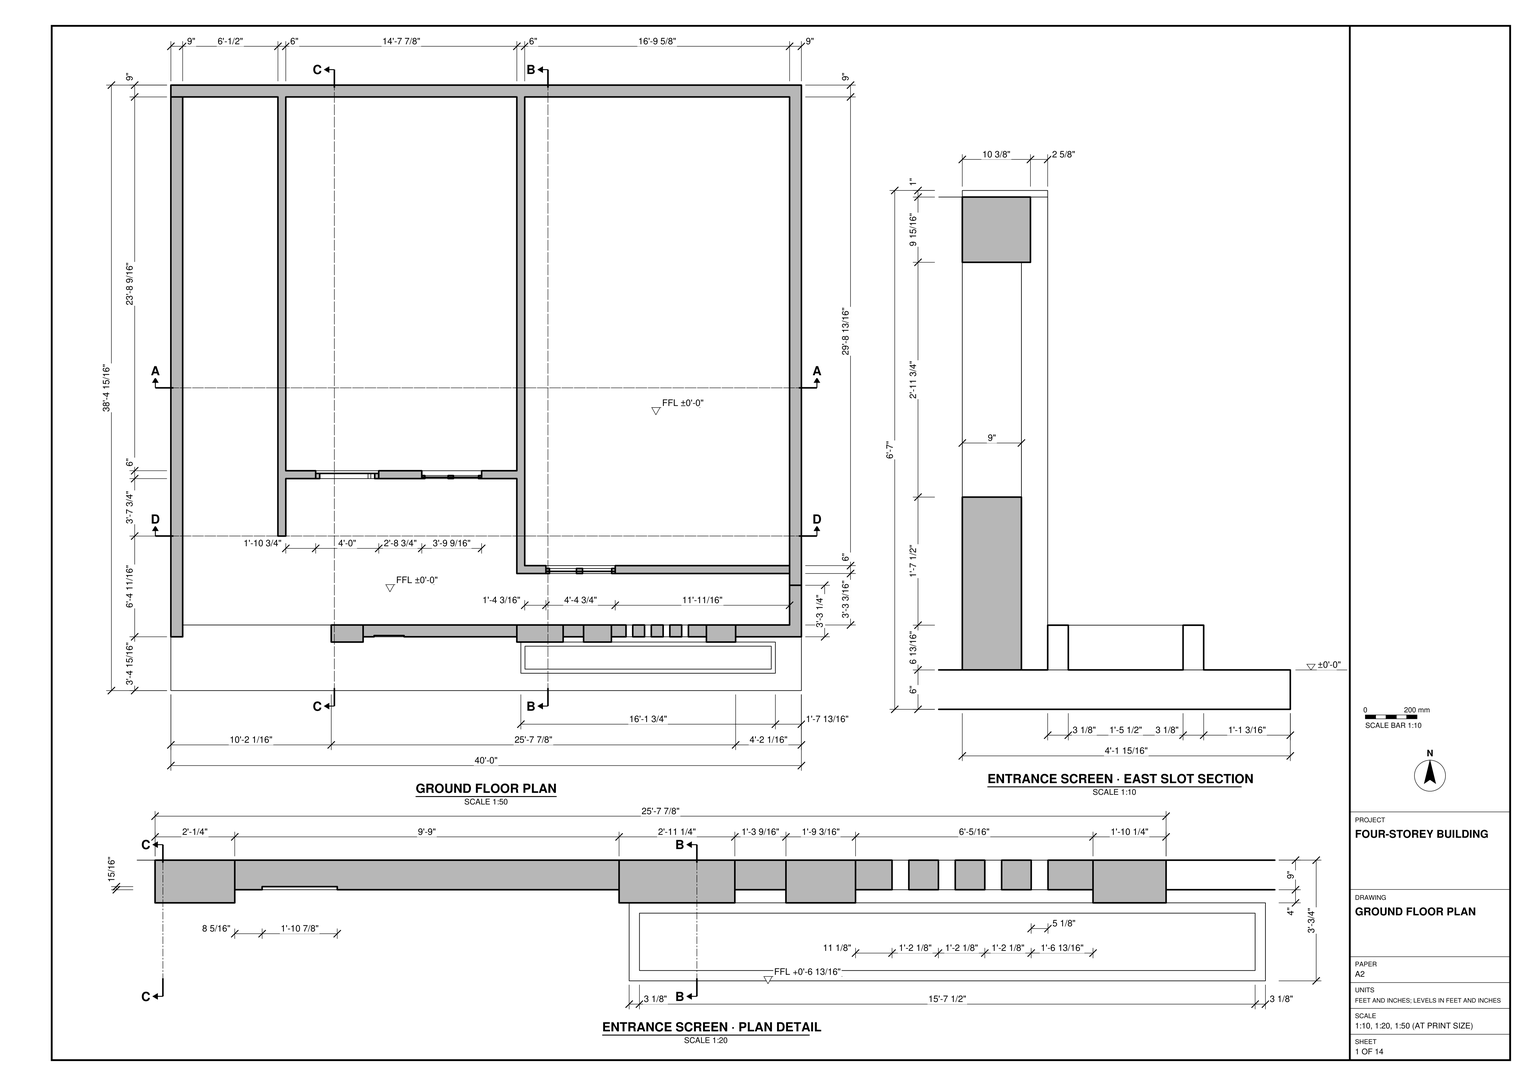
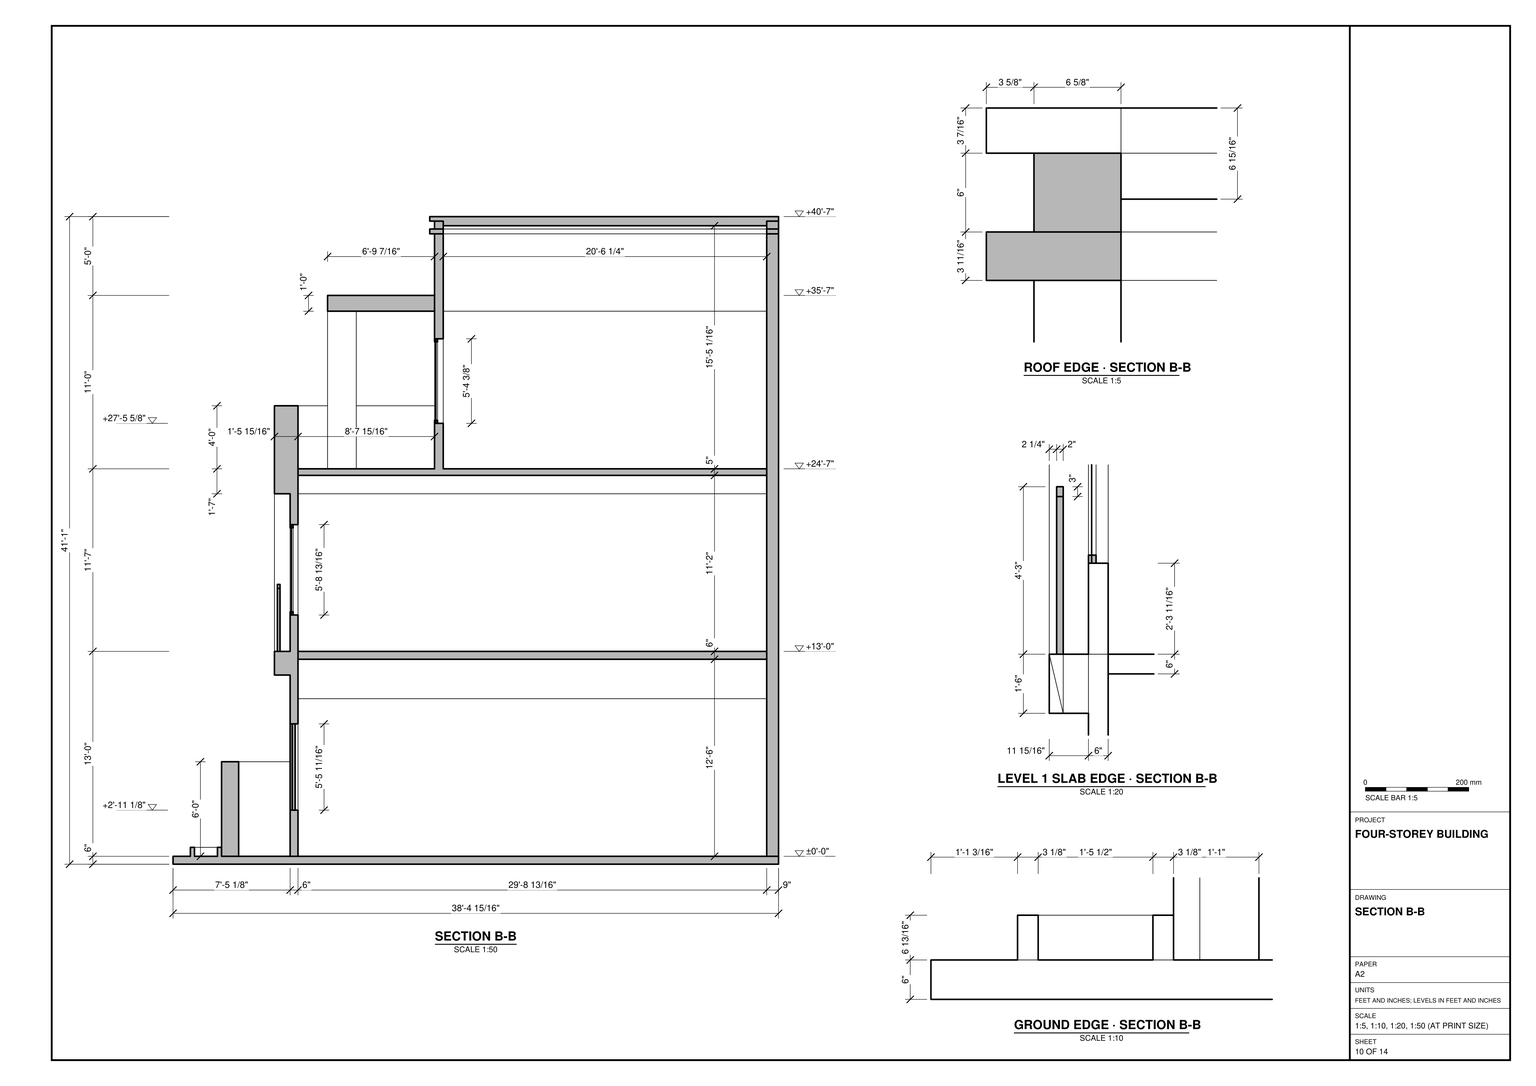
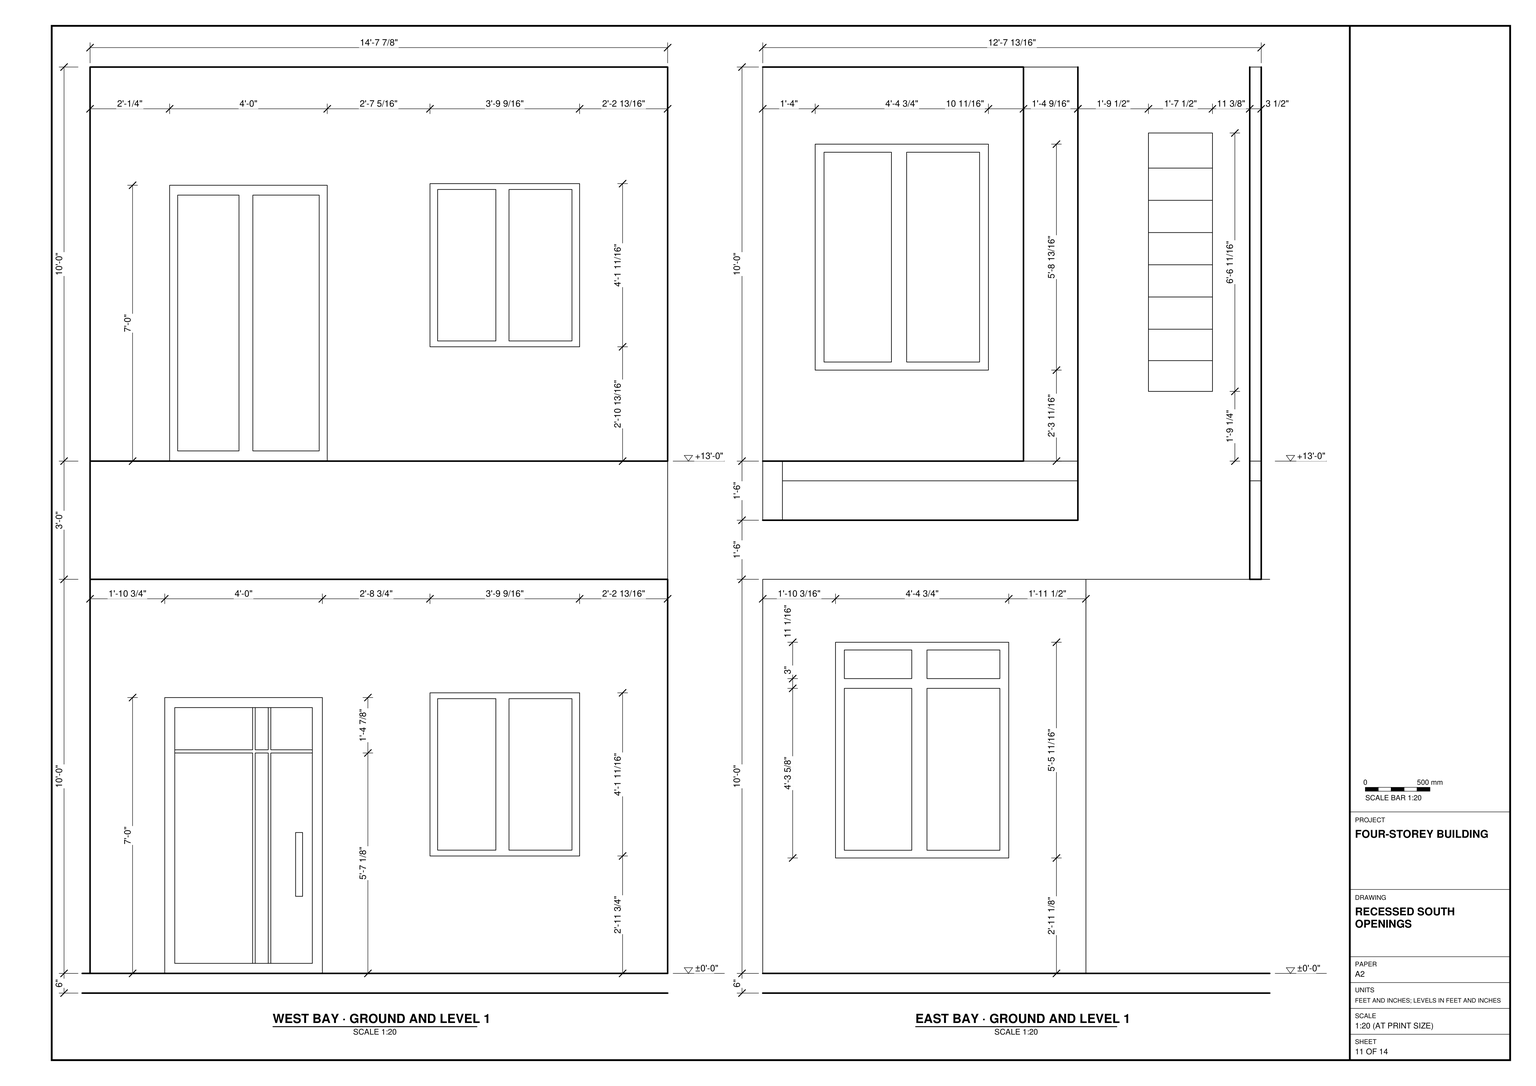
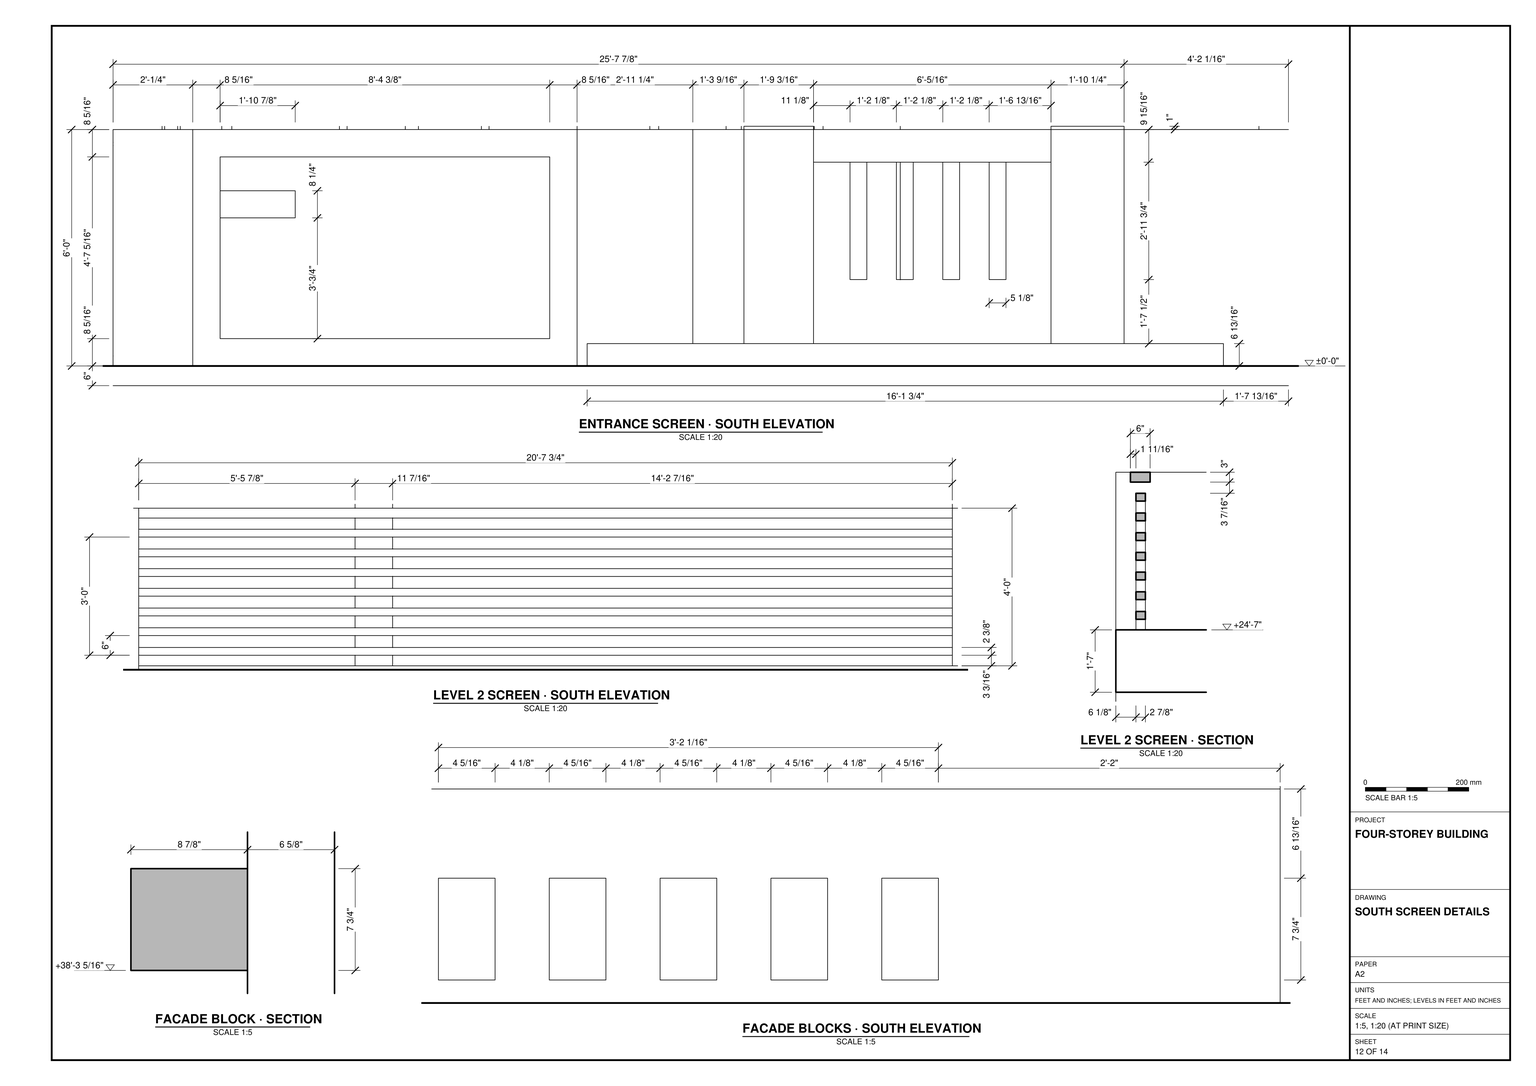
Build the four-storey building shown in task_files/diagram_01.pdf in SketchUp. Work in feet and inches. The overall model is 40'-0" wide, 38'-4 15/16" deep and 41'-1" high, measured from the underside of the ground slab to the top of the roof edge. Use the levels ±0'-0", +13'-0", +24'-7" and +35'-7" relative to the ground floor.

Use the plans to lay out the perimeter walls, internal divisions and recessed south bays. Follow the wall thicknesses shown, including the 9" perimeter walls and 6" dividing walls on the ground floor. Model the floor slabs, changes in slab edge, upper setbacks and flat roof profiles from the sections. At the south entrance, distinguish the slotted screen and low rectangular border from the door and window walls behind them. Use the enlarged opening elevations for the frames, pane divisions, heads and sills. Follow the plans and sections for stairs, built-in joinery and main furniture wherever shown.

Keep shell elements such as walls, slabs and roofs in separate groups or components. Group each furniture or joinery piece separately and use components for repeated parts. Decor and loose items, where shown, may be represented by any suitable library component. Save one SketchUp model as output_files/four_storey_building_with_its_recessed_south_entrance.skp.

# SketchUp Ruby script. Lengths in inches.
U = 1.inch
M = Sketchup.active_model
def pt(a) = Geom::Point3d.new(a.map { |v| v * U })
def face(e, loops, mat)
  f = e.add_face(loops[0].map { |a| pt(a) })
  loops[1..].each { |l| e.add_face(l.map { |a| pt(a) }).erase! }
  f.material = f.back_material = mat if mat
  f
end
# faces: each face lists its corners as indices into pts; further lists are holes
def faces(e, pts, list, mat = nil) = list.each { |f| face(e, (f[0].is_a?(Array) ? f : [f]).map { |l| l.map { |i| pts[i] } }, mat) }
# xy, xz, yz: faces in a plane at the given z, y or x. An outline is a flat list of corners, or four numbers for a rectangle; further outlines are holes
def ring(l) = l.size == 4 ? [[l[0], l[1]], [l[2], l[1]], [l[2], l[3]], [l[0], l[3]]] : l.each_slice(2).to_a
def flat(e, list, mat, &to3) = list.each { |f| face(e, (f[0].is_a?(Array) ? f : [f]).map { |l| ring(l).map { |u, v| to3.(u, v) } }, mat) }
def xy(e, z, list, mat = nil) = flat(e, list, mat) { |x, y| [x, y, z] }
def xz(e, y, list, mat = nil) = flat(e, list, mat) { |x, z| [x, y, z] }
def yz(e, x, list, mat = nil) = flat(e, list, mat) { |y, z| [x, y, z] }
def lines(e, pts, list) = list.each { |a, b| e.add_line(pt(pts[a]), pt(pts[b])) }
# prism: a flat outline (further loops are holes) pulled along v
def prism(e, loops, v, mat = nil)
  f = face(e, loops, mat); d = Geom::Vector3d.new(v.map { |x| x * U })
  f.pushpull(f.normal.samedirection?(d) ? d.length : -d.length)
end
def box(e, o, s, mat = nil) = prism(e, [[o, [o[0] + s[0], o[1], o[2]], [o[0] + s[0], o[1] + s[1], o[2]], [o[0], o[1] + s[1], o[2]]]], [0, 0, s[2]], mat)
def at(x, y, z, deg = 0) = Geom::Transformation.translation(pt([x, y, z])) * Geom::Transformation.rotation(ORIGIN, Z_AXIS, deg.degrees)
def axes(o, x, y, z) = Geom::Transformation.new([*x, 0, *y, 0, *z, 0, *pt(o).to_a, 1])
def part(name) = M.definitions.add(name)
# library, detail: a bought-in or finely detailed component or shape, given as its bounding box
def library(name, o, s) = part(name).tap { |d| box(d.entities, o, s) }
def detail(e, o, s) = box(e.add_group.entities, o, s)
def put(e, d, t, mat = nil) = e.add_instance(d, t).tap { |i| i.material = mat if mat }
def group(e, t, mat = nil) = e.add_group.tap { |g| g.transformation = t; g.material = mat if mat }.entities
root = M.entities
M.materials.add("[0012_Bisque]").color = [255, 228, 196]
M.materials.add("[0132_LightGray]").color = [169, 169, 169]
M.materials.add("[Blacktop Old 02]").color = [143, 145, 145]
M.materials.add("[Color A08]").color = [102, 0, 0]
M.materials.add("[Color C01]").color = [255, 229, 204]
M.materials.add("[Color C03]").color = [255, 178, 101]
M.materials.add("[Color C05]").color = [255, 29, 0]
M.materials.add("[Color C06]").color = [217, 132, 71]
M.materials.add("[Color C07]").color = [153, 76, 0]
M.materials.add("[Color C08]").color = [65, 44, 0]
M.materials.add("[Color C08]1").color = [102, 51, 0]
M.materials.add("[Grass Dark Green]").color = [106, 157, 55]
M.materials.add("[Metal Corrugated Shiny]").color = [193, 193, 152]
M.materials.add("[Metal Embossed]").color = [0, 0, 0]
M.materials.add("[Metal Silver]").color = [234, 233, 238]
M.materials.add("[Pavers with Grass Herringbone]").color = [197, 201, 190]
M.materials.add("[Polished Concrete New]").color = [200, 200, 203]
M.materials.add("[Stone Brushed Khaki]").color = [226, 169, 133]
M.materials.add("[Stone Coursed Rough]").color = [165, 160, 130]
M.materials.add("[Stone Flagstone Ashlar]").color = [145, 113, 102]
M.materials.add("[Stone Flagstone Ashlar]1").color = [175, 116, 102]
M.materials.add("[Translucent Glass Blue]").color = [100, 143, 235]
M.materials["[Translucent Glass Blue]"].alpha = 0.5
M.materials.add("[Translucent Glass Gray]").color = [128, 128, 128]
M.materials["[Translucent Glass Gray]"].alpha = 0.5
M.materials.add("[Wood Floor Parquet]").color = [145, 89, 39]
M.materials.add("[Wood Floor]").color = [155, 105, 61]
M.materials.add("[Wood Veneer 01]").color = [120, 70, 37]
c1 = part("Group\#2")
xy(c1.entities,0,[[0,0,37.5,1.9375],[0,1.9375,37.5,4.625]],"[Color C08]")
xy(c1.entities,1.92,[[1.92,0,16.51,1.9375],[19.8,0,35.58,1.9375],[1.92,1.9375,16.51,4.625],[19.8,1.9375,35.58,4.625]],"[Color C08]")
xy(c1.entities,51.65,[[1.92,0,16.51,1.9375],[19.8,0,35.58,1.9375],[1.92,1.9375,16.51,4.625],[19.8,1.9375,35.58,4.625]],"[Color C08]")
xy(c1.entities,53.5625,[[0,0,37.5,1.9375],[0,1.9375,37.5,4.625]],"[Color C08]")
xz(c1.entities,0,[[[0,0,37.5,53.5625],[19.8,1.92,35.58,51.65],[1.92,1.92,16.51,51.65]]],"[Color C08]")
xz(c1.entities,1.9375,[[[0,0,37.5,53.5625],[19.8,1.92,35.58,51.65],[1.92,1.92,16.51,51.65]]])
xz(c1.entities,1.9375,[[1.92,1.92,16.51,51.65],[19.8,1.92,35.58,51.65]],"[Translucent Glass Gray]")
xz(c1.entities,4.625,[[[0,0,37.5,53.5625],[19.8,1.92,35.58,51.65],[1.92,1.92,16.51,51.65]]],"[Color C08]")
yz(c1.entities,0,[[0,0,1.9375,53.5625],[1.9375,0,4.625,53.5625]],"[Color C08]")
yz(c1.entities,1.92,[[0,1.92,1.9375,51.65],[1.9375,1.92,4.625,51.65]],"[Color C08]")
yz(c1.entities,16.51,[[0,1.92,1.9375,51.65],[1.9375,1.92,4.625,51.65]],"[Color C08]")
yz(c1.entities,19.8,[[0,1.92,1.9375,51.65],[1.9375,1.92,4.625,51.65]],"[Color C08]")
yz(c1.entities,35.58,[[0,1.92,1.9375,51.65],[1.9375,1.92,4.625,51.65]],"[Color C08]")
yz(c1.entities,37.5,[[0,0,1.9375,53.5625],[1.9375,0,4.625,53.5625]],"[Color C08]")
xy(root,0,[[0,0,480,460.9375]],"[Polished Concrete New]")
xy(root,6,[[122.07,36.9375,146.35,49.9375],[263.375,36.9375,298.62,49.9375],[298.62,36.9375,314.18,40.9375],[314.18,36.9375,335.37,49.9375],[335.37,36.9375,407.6875,40.9375],
  [407.6875,36.9375,429.9375,49.9375],[0,40.9375,9,451.9375],[146.35,40.9375,263.375,49.9375],[298.62,40.9375,314.18,49.9375],[335.37,40.9375,407.6875,49.9375],
  [429.9375,40.9375,429.9375,49.9375,471,49.9375,471,80.1875,480,80.1875,480,40.9375],[471,80.1875,480,460.9375],[263.375,89.125,263.375,161.375,158.24,161.375,158.24,167.375,263.375,167.375,263.375,451.9375,87.5,451.9375,87.5,167.375,110.24,167.375,110.24,161.375,81.5,161.375,81.5,451.9375,0,451.9375,0,460.9375,269.375,460.9375,269.375,95.125,471,95.125,471,89.125],[269.375,95.125,471,451.9375],[81.5,117.625,87.5,161.375],
  [87.5,167.375,263.375,451.9375],[269.375,451.9375,471,460.9375]])
xy(root,6,[[9,49.9375,471,49.9375,471,89.125,263.375,89.125,263.375,161.375,158.24,161.375,158.24,167.375,110.24,167.375,110.24,161.375,87.5,161.375,87.5,117.625,81.5,117.625,81.5,451.9375,9,451.9375]],"[Blacktop Old 02]")
xy(root,6,[[269.58,16.33,457.05,33.8]],"[Grass Dark Green]")
xy(root,6,[[0,0,480,0,480,40.9375,429.9375,40.9375,429.9375,36.9375,460.19,36.9375,460.19,13.1875,266.44,13.1875,266.44,36.9375,263.375,36.9375,263.375,40.9375,146.35,40.9375,146.35,36.9375,122.07,36.9375,122.07,49.9375,9,49.9375,9,40.9375,0,40.9375]],"[Pavers with Grass Herringbone]")
xy(root,12.8125,[[[266.44,13.1875,460.19,36.9375],[269.58,16.33,457.05,33.8]]],"[Stone Brushed Khaki]")
xy(root,32.3125,[[346.48,40.9375,351.61,49.9375],[360.61,40.9375,365.73,49.9375],[374.73,40.9375,379.86,49.9375],[388.86,40.9375,393.98,49.9375]],"[0012_Bisque]")
xy(root,41.15,[[285.53,89.125,338.28,95.125]])
xy(root,41.75,[[191.01,161.375,236.57,167.375]])
xy(root,51.11,[[154.68,40.9375,177.55,41.875]],"[Wood Veneer 01]")
xy(root,59.36,[[154.68,40.9375,177.55,41.875]],"[Wood Veneer 01]")
xy(root,68.0625,[[346.48,39.5625,351.61,49.9375],[360.61,39.5625,365.73,49.9375],[374.73,39.5625,379.86,49.9375],[388.86,39.5625,393.98,49.9375],[335.37,40.9375,346.48,49.9375],
  [351.61,40.9375,360.61,49.9375],[365.73,40.9375,374.73,49.9375],[379.86,40.9375,388.86,49.9375],[393.98,40.9375,407.6875,49.9375]])
xy(root,68.0625,[[335.37,39.5625,346.48,40.9375],[351.61,39.5625,360.61,40.9375],[365.73,39.5625,374.73,40.9375],[379.86,39.5625,388.86,40.9375],[393.98,39.5625,407.6875,40.9375]],"[Color C03]")
xy(root,78,[[314.18,36.9375,335.37,49.9375],[407.6875,36.9375,429.9375,49.9375]])
xy(root,78,[[0,40.9375,9,451.9375]],"[Color C01]")
xy(root,78,[[335.37,39.5625,407.6875,49.9375]],"[Color C03]")
xy(root,78,[[122.07,36.9375,146.35,49.9375],[298.62,40.9375,314.18,49.9375],[429.9375,40.9375,480,40.9375,480,80.1875,471,80.1875,471,49.9375,429.9375,49.9375]],"[Stone Coursed Rough]")
xy(root,78,[[263.375,36.9375,298.62,49.9375]],"[Wood Floor]")
xy(root,78,[[146.35,40.9375,263.375,49.9375]],"[Wood Veneer 01]")
xy(root,79,[[314.18,36.9375,335.37,49.9375],[407.6875,36.9375,429.9375,49.9375]],"[0132_LightGray]")
xy(root,90,[[110.24,161.375,158.24,167.375]])
xy(root,91.4375,[[191.01,161.375,236.57,167.375]])
xy(root,106.83,[[285.53,89.125,338.28,95.125]])
xy(root,126,[[411.67,86.625,415.17,89.125]],"[Color C01]")
xy(root,126,[[0,89.125,0,451.9375,81.5,451.9375,81.5,117.625,87.5,117.625,87.5,161.375,263.375,161.375,263.375,89.125]],"[Color C07]")
xy(root,144,[[0,77.1875,218.47,89.125]],"[Color C03]")
xy(root,144,[[218.47,77.1875,359.34,89.125]],"[Color C07]")
xy(root,156,[[269.375,95.125,471,451.9375],[87.5,167.375,263.375,451.9375]])
xy(root,162,[[15.625,77.1875,342.78,79.4375],[15.625,79.4375,342.78,81.4375],[269.375,95.125,471,451.9375],[111.72,161.375,159.72,167.375],[87.5,167.375,263.375,451.9375]])
xy(root,162,[[15.625,81.4375,342.78,81.4375,342.78,89.125,263.375,89.125,263.375,161.375,87.5,161.375,87.5,117.625,81.5,117.625,81.5,451.9375,15.625,451.9375]],"[Blacktop Old 02]")
xy(root,189.71,[[279.34,89.125,332.09,95.125]])
xy(root,196.8125,[[191.01,161.375,236.57,167.375]])
xy(root,210,[[15.625,79.4375,342.78,81.4375]],"[Metal Silver]")
xy(root,213,[[15.625,79.4375,342.78,81.4375]],"[Metal Silver]")
xy(root,246,[[111.72,161.375,159.72,167.375]])
xy(root,246.5,[[191.01,161.375,236.57,167.375]])
xy(root,258.52,[[279.34,89.125,332.09,95.125]])
xy(root,282,[[15.625,77.1875,15.625,117.625,87.5,117.625,87.5,161.375,263.375,161.375,263.375,77.1875],[263.375,77.1875,342.78,89.125]],"[Color C07]")
xy(root,291.6875,[[87.5,167.375,263.375,451.9375]])
xy(root,295,[[15.625,117.625,81.5,451.9375]],"[0012_Bisque]")
xy(root,296,[[269.375,95.125,471,451.9375]])
xy(root,301,[[81.5,117.625,87.5,139.5],[87.5,117.625,92.9375,139.5],[269.375,205.6875,471,451.9375],[81.5,411.95,92.9375,451.9375]])
xy(root,301,[[15.625,77.1875,263.375,87.625],[[15.625,87.625,263.375,87.625,263.375,95.125,471,95.125,471,117.625,473.625,117.625,473.625,185.0625,348.375,185.0625,348.375,199.0625,263.375,199.0625,263.375,451.9375,92.9375,451.9375,92.9375,411.95,81.5,411.95,81.5,451.9375,15.625,451.9375],[81.5,117.625,92.9375,139.5]]],"[Blacktop Old 02]")
xy(root,304.21,[[15.625,83.31,263.375,86.18]],"[Metal Embossed]")
xy(root,306.59,[[15.625,83.31,263.375,86.18]],"[Metal Embossed]")
xy(root,310.21,[[15.625,83.31,263.375,86.18]],"[Metal Embossed]")
xy(root,312.59,[[15.625,83.31,263.375,86.18]],"[Metal Embossed]")
xy(root,316.21,[[15.625,83.31,263.375,86.18]],"[Metal Embossed]")
xy(root,318.59,[[15.625,83.31,263.375,86.18]],"[Metal Embossed]")
xy(root,322.21,[[15.625,83.31,263.375,86.18]],"[Metal Embossed]")
xy(root,324.59,[[15.625,83.31,263.375,86.18]],"[Metal Embossed]")
xy(root,328.21,[[15.625,83.31,263.375,86.18]],"[Metal Embossed]")
xy(root,330.59,[[15.625,83.31,263.375,86.18]],"[Metal Embossed]")
xy(root,334.21,[[15.625,83.31,263.375,86.18]],"[Metal Embossed]")
xy(root,335.61,[[279.78,199.0625,330.65,205.6875]])
xy(root,336.59,[[15.625,83.31,263.375,86.18]],"[Metal Embossed]")
xy(root,340.21,[[15.625,83.31,263.375,86.18]],"[Metal Embossed]")
xy(root,342.59,[[15.625,83.31,263.375,86.18]],"[Metal Embossed]")
xy(root,346,[[15.625,81.625,263.375,87.625]],"[Metal Embossed]")
xy(root,349,[[0,77.1875,15.625,77.1875,15.625,451.9375,263.375,451.9375,263.375,460.9375,0,460.9375],[263.375,77.1875,359.34,77.1875,359.34,89.125,411.67,89.125,411.67,86.625,415.17,86.625,415.17,89.125,471,89.125,471,80.1875,480,80.1875,480,117.625,471,117.625,471,95.125,263.375,95.125]],"[Color C01]")
xy(root,349,[[15.625,81.625,263.375,87.625]],"[Metal Embossed]")
xy(root,399.99,[[279.78,199.0625,330.65,205.6875]])
xy(root,421,[[348.375,185.0625,473.625,199.0625]])
xy(root,421,[[[92.9375,117.625,92.9375,139.5,81.5,139.5,81.5,411.95,92.9375,411.95,92.9375,451.9375,263.375,451.9375,263.375,199.0625,348.375,199.0625,348.375,185.0625,473.625,185.0625,473.625,117.625],[121.07,215.73,134.32,377.23],[169.89,215.73,183.14,377.23],[146.07,215.73,159.32,377.23],[193.82,215.73,207.07,377.23]]],"[0012_Bisque]")
xy(root,433,[[[81.5,117.625,480,117.625,480,199.0625,263.375,199.0625,263.375,451.9375,81.5,451.9375],[121.07,215.73,134.32,377.23],[146.07,215.73,159.32,377.23],[169.89,215.73,183.14,377.23],[193.82,215.73,207.07,377.23]]],"[0012_Bisque]")
xy(root,465.33,[[415.92,190.1875,420.24,199.0625],[424.36,190.1875,428.67,199.0625],[432.8,190.1875,437.11,199.0625],[441.24,190.1875,445.55,199.0625],[449.67,190.1875,453.99,199.0625]],"[Color C01]")
xy(root,473.08,[[415.92,190.1875,420.24,199.0625],[424.36,190.1875,428.67,199.0625],[432.8,190.1875,437.11,199.0625],[441.24,190.1875,445.55,199.0625],[449.67,190.1875,453.99,199.0625]],"[Color C01]")
xy(root,479.875,[[[263.375,199.0625,480,460.9375],[269.375,205.6875,471,451.9375]]])
xy(root,479.875,[[258.375,195.4375,258.375,460.9375,263.375,460.9375,263.375,199.0625,480,199.0625,480,195.4375]],"[Color C08]1")
xy(root,483.5625,[[[263.375,199.0625,480,460.9375],[269.375,205.6875,471,451.9375]]])
xy(root,483.5625,[[258.375,195.4375,480,195.4375,480,199.0625,263.375,199.0625,263.375,460.9375,258.375,460.9375]],"[Color C08]1")
xy(root,486.0625,[[269.375,205.6875,471,451.9375]])
xy(root,489.5625,[[[263.375,199.0625,480,460.9375],[269.375,205.6875,471,451.9375]]])
xy(root,489.5625,[[258.375,195.4375,258.375,460.9375,263.375,460.9375,263.375,199.0625,480,199.0625,480,195.4375]],"[Color C08]1")
xy(root,493,[[258.375,195.4375,480,460.9375]],"[Color C08]1")
xz(root,0,[[0,0,480,6]],"[Polished Concrete New]")
xz(root,13.1875,[[266.44,6,460.19,12.8125]],"[Stone Brushed Khaki]")
xz(root,16.33,[[269.58,6,457.05,12.8125]])
xz(root,33.8,[[269.58,6,457.05,12.8125]],"[Stone Brushed Khaki]")
xz(root,36.9375,[[266.44,6,298.62,12.8125],[298.62,6,314.18,12.8125],[314.18,6,335.37,12.8125],[335.37,6,407.6875,12.8125],[407.6875,6,429.9375,12.8125],
  [429.9375,6,460.19,12.8125]])
xz(root,36.9375,[[314.18,12.8125,335.37,78],[407.6875,12.8125,429.9375,78]],"[0012_Bisque]")
xz(root,36.9375,[[314.18,78,335.37,79],[407.6875,78,429.9375,79]],"[0132_LightGray]")
xz(root,36.9375,[[122.07,6,146.35,78]],"[Stone Coursed Rough]")
xz(root,36.9375,[[263.375,6,266.44,6,266.44,12.8125,298.62,12.8125,298.62,78,263.375,78]],"[Wood Floor]")
xz(root,39.5625,[[335.37,68.0625,407.6875,78]],"[Color C03]")
xz(root,40.9375,[[335.37,6,407.6875,6,407.6875,68.0625,393.98,68.0625,393.98,32.3125,388.86,32.3125,388.86,68.0625,379.86,68.0625,379.86,32.3125,374.73,32.3125,374.73,68.0625,365.73,68.0625,365.73,32.3125,360.61,32.3125,360.61,68.0625,351.61,68.0625,351.61,32.3125,346.48,32.3125,346.48,68.0625,335.37,68.0625]],"[0012_Bisque]")
xz(root,40.9375,[[0,6,9,78]],"[Color C01]")
xz(root,40.9375,[[298.62,6,314.18,78],[429.9375,6,480,78]],"[Stone Coursed Rough]")
xz(root,40.9375,[[154.68,14.33,255.05,14.33,255.05,69.67,154.68,69.67,154.68,59.36,177.55,59.36,177.55,51.11,154.68,51.11]],"[Wood Floor]")
xz(root,40.9375,[[[146.35,6,263.375,78],[154.68,14.33,255.05,69.67]]],"[Wood Veneer 01]")
xz(root,41.875,[[154.68,51.11,177.55,59.36]],"[Wood Veneer 01]")
xz(root,49.9375,[[335.37,6,335.37,68.0625,346.48,68.0625,346.48,32.3125,351.61,32.3125,351.61,68.0625,360.61,68.0625,360.61,32.3125,365.73,32.3125,365.73,68.0625,374.73,68.0625,374.73,32.3125,379.86,32.3125,379.86,68.0625,388.86,68.0625,388.86,32.3125,393.98,32.3125,393.98,68.0625,407.6875,68.0625,407.6875,6]],"[0012_Bisque]")
xz(root,49.9375,[[314.18,78,335.37,79],[407.6875,78,429.9375,79]],"[0132_LightGray]")
xz(root,49.9375,[[314.18,6,335.37,78],[407.6875,6,429.9375,78]],"[Color C01]")
xz(root,49.9375,[[335.37,68.0625,407.6875,78]],"[Color C03]")
xz(root,49.9375,[[122.07,6,146.35,78],[298.62,6,314.18,78],[429.9375,6,471,78]],"[Stone Coursed Rough]")
xz(root,49.9375,[[263.375,6,298.62,78]],"[Wood Floor]")
xz(root,49.9375,[[146.35,6,263.375,78]],"[Wood Veneer 01]")
xz(root,77.1875,[[263.375,301,359.34,349]],"[Color C01]")
xz(root,77.1875,[[15.625,144,218.47,162]],"[Color C03]")
xz(root,77.1875,[[0,144,15.625,349]],"[Color C06]")
xz(root,77.1875,[[218.47,144,359.34,144,359.34,301,15.625,301,15.625,282,342.78,282,342.78,162,218.47,162]],"[Color C07]")
xz(root,79.4375,[[15.625,210,342.78,213]],"[Metal Silver]")
xz(root,79.4375,[[15.625,162,342.78,210]],"[Translucent Glass Gray]")
xz(root,80.1875,[[471,6,480,78]])
xz(root,80.1875,[[471,78,480,349]],"[Color C06]")
xz(root,81.4375,[[15.625,210,342.78,213]],"[Metal Silver]")
xz(root,81.4375,[[15.625,162,342.78,210]],"[Translucent Glass Gray]")
xz(root,81.625,[[15.625,346,263.375,349]],"[Metal Embossed]")
xz(root,83.31,[[15.625,304.21,263.375,306.59],[15.625,310.21,263.375,312.59],[15.625,316.21,263.375,318.59],[15.625,322.21,263.375,324.59],[15.625,328.21,263.375,330.59],
  [15.625,334.21,263.375,336.59],[15.625,340.21,263.375,342.59]],"[Metal Embossed]")
xz(root,86.18,[[15.625,304.21,263.375,306.59],[15.625,310.21,263.375,312.59],[15.625,316.21,263.375,318.59],[15.625,322.21,263.375,324.59],[15.625,328.21,263.375,330.59],
  [15.625,334.21,263.375,336.59],[15.625,340.21,263.375,342.59]],"[Metal Embossed]")
xz(root,86.625,[[411.67,126,415.17,349]],"[Color C01]")
xz(root,87.625,[[15.625,346,263.375,349]],"[Metal Embossed]")
xz(root,89.125,[[[82.03,126,411.67,126,411.67,349,359.34,349,359.34,144,82.03,144],[380.82,183.23,400.32,261.92]],[[263.375,162,342.78,282],[279.34,189.71,332.09,258.52]]],"[0012_Bisque]")
xz(root,89.125,[[380.82,192.6,400.32,202.16],[380.82,211.98,400.32,221.79],[380.82,231.6,400.32,241.41],[380.82,251.23,400.32,261.92]],"[Color A08]")
xz(root,89.125,[[[263.375,6,361.79,126],[285.53,41.15,338.28,106.83]]],"[Color C01]")
xz(root,89.125,[[0,126,82.03,144],[380.82,183.23,400.32,192.6],[380.82,202.16,400.32,211.98],[380.82,221.79,400.32,231.6],[380.82,241.41,400.32,251.23]],"[Color C03]")
xz(root,89.125,[[415.17,126,471,349]],"[Color C06]")
xz(root,89.125,[[361.79,6,471,126]],"[Stone Flagstone Ashlar]")
xz(root,95.125,[[[269.375,6,471,126],[285.53,41.15,338.28,106.83]],[269.375,126,471,156],[269.375,156,418.875,162],[418.875,156,437.9375,162],[437.9375,156,471,162],
  [[269.375,162,471,282],[279.34,189.71,332.09,258.52]],[269.375,282,471,296],[269.375,296,287.5,301]])
xz(root,95.125,[[263.375,301,269.375,349],[269.375,301,287.5,349],[287.5,301,471,349]],"[Color C01]")
xz(root,117.625,[[81.5,126,87.5,162],[15.625,282,81.5,295],[81.5,282,87.5,301]])
xz(root,117.625,[[81.5,6,87.5,126],[81.5,162,87.5,282],[81.5,301,92.9375,301,92.9375,421,473.625,421,473.625,349,480,349,480,433,81.5,433]],"[0012_Bisque]")
xz(root,117.625,[[471,301,473.625,349]],"[Color C01]")
xz(root,139.5,[[81.5,301,92.9375,421]],"[Color C01]")
xz(root,161.375,[[87.5,126,263.375,162]])
xz(root,161.375,[[[87.5,6,110.24,6,110.24,90,158.24,90,158.24,6,263.375,6,263.375,126,87.5,126],[191.01,41.75,236.57,91.4375]],[[87.5,162,111.72,162,111.72,246,159.72,246,159.72,162,263.375,162,263.375,282,87.5,282],[191.01,196.8125,236.57,246.5]]],"[0012_Bisque]")
xz(root,167.375,[[[87.5,6,87.5,126,263.375,126,263.375,6,158.24,6,158.24,90,110.24,90,110.24,6],[191.01,41.75,236.57,91.4375]],[87.5,126,263.375,156],[87.5,156,111.72,162],[111.72,156,159.72,162],[159.72,156,205.18,162],
  [205.18,156,211.55,162],[211.55,156,263.375,162],[[87.5,162,87.5,282,263.375,282,263.375,162,159.72,162,159.72,246,111.72,246,111.72,162],[191.01,196.8125,236.57,246.5]],[87.5,282,263.375,291.6875]])
xz(root,185.0625,[[348.375,301,473.625,421]],"[Stone Flagstone Ashlar]")
xz(root,190.1875,[[415.92,465.33,420.24,473.08],[424.36,465.33,428.67,473.08],[432.8,465.33,437.11,473.08],[441.24,465.33,445.55,473.08],[449.67,465.33,453.99,473.08]],"[Color C01]")
xz(root,195.4375,[[258.375,479.875,480,483.5625],[258.375,489.5625,480,493]],"[Color C08]1")
xz(root,199.0625,[[263.375,421,473.625,433],[415.92,465.33,420.24,473.08],[424.36,465.33,428.67,473.08],[432.8,465.33,437.11,473.08],[441.24,465.33,445.55,473.08],
  [449.67,465.33,453.99,473.08]])
xz(root,199.0625,[[263.375,301,348.375,301,348.375,367.8,330.65,367.8,330.65,335.61,279.78,335.61,279.78,367.38,263.375,367.38],[263.375,483.5625,480,489.5625]],"[Color C01]")
xz(root,199.0625,[[263.375,367.38,279.78,367.38,279.78,399.99,330.65,399.99,330.65,367.8,348.375,367.8,348.375,421,263.375,421],[263.375,433,348.375,479.875]],"[Color C05]")
xz(root,199.0625,[[[348.375,433,480,479.875],[449.67,465.33,453.99,473.08],[441.24,465.33,445.55,473.08],[432.8,465.33,437.11,473.08],[424.36,465.33,428.67,473.08],[415.92,465.33,420.24,473.08]]],"[Stone Flagstone Ashlar]1")
xz(root,205.6875,[[[269.375,301,471,421],[279.78,335.61,330.65,399.99]],[269.375,421,471,479.875],[269.375,479.875,471,483.5625],[269.375,483.5625,471,486.0625],[269.375,486.0625,275.375,489.5625],
  [275.375,486.0625,471,489.5625]])
xz(root,215.73,[[121.07,421,134.32,433],[146.07,421,159.32,433],[169.89,421,183.14,433],[193.82,421,207.07,433]],"[Color C01]")
xz(root,377.23,[[121.07,421,134.32,433],[146.07,421,159.32,433],[169.89,421,183.14,433],[193.82,421,207.07,433]],"[0012_Bisque]")
xz(root,411.95,[[81.5,301,92.9375,421]],"[0012_Bisque]")
xz(root,451.9375,[[0,6,9,78],[87.5,6,263.375,126],[269.375,6,471,126],[9,126,81.5,162],[87.5,126,263.375,156],
  [269.375,126,471,156],[87.5,156,263.375,162],[269.375,156,471,162],[9,162,15.625,301],[87.5,162,263.375,282],
  [269.375,162,471,282],[87.5,282,263.375,291.6875],[269.375,282,471,296],[87.5,291.6875,263.375,301],[15.625,295,81.5,301],
  [269.375,296,471,301],[81.5,301,87.5,349],[87.5,301,92.9375,349],[269.375,301,471,421],[269.375,421,471,479.875],
  [269.375,479.875,471,483.5625],[269.375,483.5625,471,486.0625],[269.375,486.0625,471,489.5625]])
xz(root,451.9375,[[15.625,162,81.5,295]],"[0012_Bisque]")
xz(root,451.9375,[[9,6,81.5,6,81.5,126,0,126,0,78,9,78],[15.625,301,81.5,349],[92.9375,301,263.375,349],[81.5,349,81.5,433,263.375,433,263.375,421,92.9375,421,92.9375,349]],"[Color C01]")
xz(root,460.9375,[[0,6,0,349,263.375,349,263.375,301,480,301,480,6],[263.375,483.5625,480,489.5625]],"[Color C01]")
xz(root,460.9375,[[263.375,301,480,479.875]],"[Color C05]")
xz(root,460.9375,[[258.375,479.875,480,483.5625],[258.375,489.5625,480,493]],"[Color C08]1")
xz(root,460.9375,[[0,0,480,6]],"[Polished Concrete New]")
yz(root,0,[[40.9375,6,451.9375,78],[451.9375,6,451.9375,126,89.125,126,89.125,144,77.1875,144,77.1875,349,460.9375,349,460.9375,6]],"[Color C01]")
yz(root,0,[[0,0,460.9375,6]],"[Polished Concrete New]")
yz(root,9,[[40.9375,6,451.9375,78]],"[Color C01]")
yz(root,15.625,[[79.4375,162,81.4375,210],[77.1875,282,117.625,301],[117.625,295,451.9375,301],[83.31,304.21,86.18,306.59],[83.31,310.21,86.18,312.59],
  [83.31,316.21,86.18,318.59],[83.31,322.21,86.18,324.59],[83.31,328.21,86.18,330.59],[83.31,334.21,86.18,336.59],[83.31,340.21,86.18,342.59]])
yz(root,15.625,[[77.1875,162,79.4375,162,79.4375,213,81.4375,213,81.4375,162,451.9375,162,451.9375,295,117.625,295,117.625,282,77.1875,282]],"[0012_Bisque]")
yz(root,15.625,[[77.1875,301,83.31,301,83.31,342.59,86.18,342.59,86.18,301,451.9375,301,451.9375,349,87.625,349,87.625,346,81.625,346,81.625,349,77.1875,349]],"[Color C01]")
yz(root,15.625,[[83.31,301,86.18,304.21],[83.31,306.59,86.18,310.21],[83.31,312.59,86.18,316.21],[83.31,318.59,86.18,322.21],[83.31,324.59,86.18,328.21],
  [83.31,330.59,86.18,334.21],[83.31,336.59,86.18,340.21]],"[Metal Embossed]")
yz(root,15.625,[[79.4375,210,81.4375,213]],"[Metal Silver]")
yz(root,81.5,[[117.625,126,451.9375,162],[117.625,295,139.5,301],[411.95,295,451.9375,301]])
yz(root,81.5,[[117.625,6,451.9375,126],[117.625,162,451.9375,295],[117.625,301,117.625,433,451.9375,433,451.9375,301,411.95,301,411.95,421,139.5,421,139.5,301]],"[0012_Bisque]")
yz(root,87.5,[[167.375,6,451.9375,126],[117.625,126,161.375,162],[167.375,126,451.9375,156],[167.375,156,451.9375,162],[167.375,162,451.9375,282],
  [167.375,282,451.9375,291.6875]])
yz(root,87.5,[[117.625,6,161.375,126],[117.625,162,161.375,282]],"[0012_Bisque]")
yz(root,92.9375,[[117.625,301,139.5,421],[411.95,301,451.9375,421]],"[0012_Bisque]")
yz(root,110.24,[[161.375,6,167.375,90]])
yz(root,111.72,[[161.375,162,167.375,246]])
yz(root,121.07,[[215.73,421,377.23,433]],"[0012_Bisque]")
yz(root,122.07,[[36.9375,6,49.9375,78]],"[Stone Coursed Rough]")
yz(root,134.32,[[215.73,421,377.23,433]],"[0012_Bisque]")
yz(root,146.07,[[215.73,421,377.23,433]],"[0012_Bisque]")
yz(root,146.35,[[40.9375,6,49.9375,78]])
yz(root,146.35,[[36.9375,6,40.9375,78]],"[Stone Coursed Rough]")
yz(root,154.68,[[40.9375,51.11,41.875,59.36]],"[Wood Veneer 01]")
yz(root,158.24,[[161.375,6,167.375,90]])
yz(root,159.32,[[215.73,421,377.23,433]],"[0012_Bisque]")
yz(root,159.72,[[161.375,162,167.375,246]])
yz(root,169.89,[[215.73,421,377.23,433]],"[0012_Bisque]")
yz(root,177.55,[[40.9375,51.11,41.875,59.36]],"[Wood Veneer 01]")
yz(root,183.14,[[215.73,421,377.23,433]],"[0012_Bisque]")
yz(root,191.01,[[161.375,41.75,167.375,91.4375],[161.375,196.8125,167.375,246.5]])
yz(root,193.82,[[215.73,421,377.23,433]],"[0012_Bisque]")
yz(root,207.07,[[215.73,421,377.23,433]],"[0012_Bisque]")
yz(root,218.47,[[77.1875,144,81.4375,144,77.1875,162]])
yz(root,236.57,[[161.375,41.75,167.375,91.4375],[161.375,196.8125,167.375,246.5]])
yz(root,258.375,[[195.4375,479.875,460.9375,483.5625],[195.4375,489.5625,460.9375,493]],"[Color C08]1")
yz(root,263.375,[[40.9375,6,49.9375,78],[167.375,6,451.9375,126],[167.375,126,451.9375,156],[167.375,156,451.9375,162],[167.375,162,451.9375,282],
  [167.375,282,451.9375,291.6875],[83.31,299.71,86.18,301],[451.9375,301,460.9375,349],[199.0625,421,451.9375,433]])
yz(root,263.375,[[89.125,162,161.375,282]],"[0012_Bisque]")
yz(root,263.375,[[89.125,6,161.375,126],[77.1875,301,81.625,349],[87.625,301,95.125,349],[199.0625,483.5625,460.9375,489.5625]],"[Color C01]")
yz(root,263.375,[[199.0625,301,199.0625,421,451.9375,421,451.9375,433,199.0625,433,199.0625,479.875,460.9375,479.875,460.9375,349,451.9375,349,451.9375,301]],"[Color C05]")
yz(root,263.375,[[[81.625,301,87.625,346],[83.31,340.21,86.18,342.59],[83.31,334.21,86.18,336.59],[83.31,328.21,86.18,330.59],[83.31,322.21,86.18,324.59],[83.31,316.21,86.18,318.59],[83.31,310.21,86.18,312.59],[83.31,304.21,86.18,306.59]]],"[Color C08]1")
yz(root,263.375,[[83.31,304.21,86.18,306.59],[83.31,310.21,86.18,312.59],[83.31,316.21,86.18,318.59],[83.31,322.21,86.18,324.59],[83.31,328.21,86.18,330.59],
  [83.31,334.21,86.18,336.59],[83.31,340.21,86.18,342.59],[81.625,346,87.625,349]],"[Metal Embossed]")
yz(root,263.375,[[36.9375,6,40.9375,78]],"[Wood Floor]")
yz(root,266.44,[[13.1875,6,36.9375,12.8125]],"[Stone Brushed Khaki]")
yz(root,269.375,[[95.125,6,451.9375,126],[95.125,126,451.9375,156],[95.125,156,451.9375,162],[95.125,162,451.9375,282],[95.125,282,451.9375,296],
  [205.6875,301,451.9375,421],[205.6875,421,451.9375,479.875],[205.6875,479.875,451.9375,483.5625],[205.6875,483.5625,451.9375,486.0625],[205.6875,486.0625,451.9375,489.5625]])
yz(root,269.58,[[16.33,6,33.8,12.8125]],"[Stone Brushed Khaki]")
yz(root,279.34,[[89.125,189.71,95.125,258.52]])
yz(root,279.78,[[199.0625,335.61,205.6875,399.99]])
yz(root,285.53,[[89.125,41.15,95.125,106.83]])
yz(root,298.62,[[40.9375,6,49.9375,78]])
yz(root,298.62,[[36.9375,6,40.9375,78]],"[Wood Floor]")
yz(root,314.18,[[40.9375,6,49.9375,78]])
yz(root,314.18,[[36.9375,6,40.9375,78]],"[0012_Bisque]")
yz(root,314.18,[[36.9375,78,49.9375,79]],"[0132_LightGray]")
yz(root,330.65,[[199.0625,335.61,205.6875,399.99]])
yz(root,332.09,[[89.125,189.71,95.125,258.52]])
yz(root,335.37,[[40.9375,6,49.9375,68.0625],[39.5625,68.0625,49.9375,78]])
yz(root,335.37,[[36.9375,6,36.9375,78,39.5625,78,39.5625,68.0625,40.9375,68.0625,40.9375,6]],"[0012_Bisque]")
yz(root,335.37,[[36.9375,78,49.9375,79]],"[0132_LightGray]")
yz(root,338.28,[[89.125,41.15,95.125,106.83]])
yz(root,342.78,[[79.4375,162,81.4375,210]])
yz(root,342.78,[[77.1875,162,77.1875,282,89.125,282,89.125,162,81.4375,162,81.4375,213,79.4375,213,79.4375,162]],"[Color C07]")
yz(root,342.78,[[79.4375,210,81.4375,213]],"[Metal Silver]")
yz(root,346.48,[[40.9375,32.3125,49.9375,68.0625]],"[0012_Bisque]")
yz(root,348.375,[[185.0625,301,199.0625,421]],"[Stone Flagstone Ashlar]")
yz(root,351.61,[[40.9375,32.3125,49.9375,68.0625]],"[0012_Bisque]")
yz(root,359.34,[[77.1875,301,89.125,349]],"[0012_Bisque]")
yz(root,359.34,[[77.1875,144,89.125,301]],"[Color C07]")
yz(root,360.61,[[40.9375,32.3125,49.9375,68.0625]],"[0012_Bisque]")
yz(root,365.73,[[40.9375,32.3125,49.9375,68.0625]],"[0012_Bisque]")
yz(root,374.73,[[40.9375,32.3125,49.9375,68.0625]],"[0012_Bisque]")
yz(root,379.86,[[40.9375,32.3125,49.9375,68.0625]],"[0012_Bisque]")
yz(root,388.86,[[40.9375,32.3125,49.9375,68.0625]],"[0012_Bisque]")
yz(root,393.98,[[40.9375,32.3125,49.9375,68.0625]],"[0012_Bisque]")
yz(root,407.6875,[[40.9375,6,49.9375,68.0625],[39.5625,68.0625,49.9375,78]])
yz(root,407.6875,[[36.9375,6,36.9375,78,39.5625,78,39.5625,68.0625,40.9375,68.0625,40.9375,6]],"[0012_Bisque]")
yz(root,407.6875,[[36.9375,78,49.9375,79]],"[0132_LightGray]")
yz(root,411.67,[[86.625,126,89.125,349]],"[Color C01]")
yz(root,415.17,[[86.625,126,89.125,349]],"[Color C01]")
yz(root,415.92,[[190.1875,465.33,199.0625,473.08]],"[Color C01]")
yz(root,420.24,[[190.1875,465.33,199.0625,473.08]],"[Color C01]")
yz(root,424.36,[[190.1875,465.33,199.0625,473.08]],"[Color C01]")
yz(root,428.67,[[190.1875,465.33,199.0625,473.08]],"[Color C01]")
yz(root,429.9375,[[40.9375,6,49.9375,78]])
yz(root,429.9375,[[36.9375,6,40.9375,78]],"[0012_Bisque]")
yz(root,429.9375,[[36.9375,78,49.9375,79]],"[0132_LightGray]")
yz(root,432.8,[[190.1875,465.33,199.0625,473.08]],"[Color C01]")
yz(root,437.11,[[190.1875,465.33,199.0625,473.08]],"[Color C01]")
yz(root,441.24,[[190.1875,465.33,199.0625,473.08]],"[Color C01]")
yz(root,445.55,[[190.1875,465.33,199.0625,473.08]],"[Color C01]")
yz(root,449.67,[[190.1875,465.33,199.0625,473.08]],"[Color C01]")
yz(root,453.99,[[190.1875,465.33,199.0625,473.08]],"[Color C01]")
yz(root,457.05,[[16.33,6,33.8,12.8125]],"[Stone Brushed Khaki]")
yz(root,460.19,[[13.1875,6,36.9375,12.8125]],"[Stone Brushed Khaki]")
yz(root,471,[[89.125,6,95.125,126],[95.125,6,451.9375,126],[89.125,126,95.125,150],[95.125,126,451.9375,156],[89.125,150,95.125,162],
  [95.125,156,451.9375,162],[89.125,162,95.125,282],[95.125,162,451.9375,282],[95.125,282,451.9375,296],[205.6875,301,451.9375,421],
  [205.6875,421,451.9375,479.875],[205.6875,479.875,451.9375,483.5625],[205.6875,483.5625,451.9375,486.0625],[205.6875,486.0625,451.9375,489.5625]])
yz(root,471,[[95.125,301,117.625,349]],"[Color C01]")
yz(root,471,[[80.1875,6,89.125,349]],"[Color C06]")
yz(root,471,[[49.9375,6,80.1875,78]],"[Stone Coursed Rough]")
yz(root,473.625,[[117.625,301,185.0625,421]],"[Color C01]")
yz(root,480,[[80.1875,6,460.9375,6,460.9375,433,117.625,433,117.625,349,80.1875,349],[199.0625,483.5625,460.9375,489.5625]],"[Color C01]")
yz(root,480,[[199.0625,433,460.9375,479.875]],"[Color C05]")
yz(root,480,[[195.4375,479.875,460.9375,483.5625],[195.4375,489.5625,460.9375,493]],"[Color C08]1")
yz(root,480,[[0,0,460.9375,6]],"[Polished Concrete New]")
yz(root,480,[[40.9375,6,80.1875,78]],"[Stone Coursed Rough]")
p = [[269.375,451.9375,126],[269.375,460.9375,126],[263.375,161.375,282],[263.375,161.375,301],[87.5,161.375,301],[87.5,161.375,282],
  [9,451.9375,162],[0,451.9375,162],[93.5,167.375,301],[93.5,167.375,291.6875],[263.375,167.375,291.6875],[263.375,167.375,301],
  [81.5,161.375,295],[81.5,161.375,301],[275.375,205.6875,493],[275.375,205.6875,489.5625],[269.375,205.6875,493],[269.375,205.6875,489.5625],
  [471,205.6875,493],[471,205.6875,489.5625],[471,451.9375,493],[471,451.9375,489.5625],[9,451.9375,301],[0,451.9375,301],
  [263.375,89.125,144],[263.375,89.125,162],[218.47,81.4375,162],[218.47,81.4375,144],[473.625,117.625,301],[480,117.625,301]]
lines(root,p,[[0,1],[2,3],[4,5],[6,7],[8,9],[10,11],[12,13],[14,15],[16,17],[18,19],[20,21],[22,23],
  [24,25],[26,27],[28,29]])
g1 = group(root,at(110.24,161.375,6))
xy(g1,0,[[0,0,48,3.9375]],"[Wood Floor Parquet]")
xy(g1,3.05,[[3.05,0,44.95,3.9375]],"[Wood Floor Parquet]")
xy(g1,23.47,[[39.85,0,41.97,3.9375]],"[Metal Corrugated Shiny]")
xy(g1,42.9,[[39.85,0,41.97,3.9375]],"[Metal Corrugated Shiny]")
xy(g1,80.95,[[3.05,0,44.95,3.9375]],"[Wood Floor Parquet]")
xy(g1,84,[[0,0,48,3.9375]],"[Wood Floor Parquet]")
xz(g1,0,[[39.85,23.47,41.97,42.9]],"[Metal Corrugated Shiny]")
xz(g1,0,[[[0,0,48,84],[3.05,3.05,44.95,80.95]]],"[Wood Floor Parquet]")
xz(g1,3.9375,[[39.85,23.47,41.97,42.9]])
xz(g1,3.9375,[[26.77,3.05,27.55,3.05,27.55,67.12,31.52,67.12,31.52,3.05,32.3,3.05,32.3,67.12,44.95,67.12,44.95,68.09,32.3,68.09,32.3,80.95,31.52,80.95,31.52,68.09,27.55,68.09,27.55,80.95,26.77,80.95,26.77,68.09,3.05,68.09,3.05,67.12,26.77,67.12]],"[0012_Bisque]")
xz(g1,3.9375,[[[0,0,48,84],[3.05,3.05,44.95,80.95]],[3.05,3.05,26.77,67.12],[27.55,3.05,31.52,67.12],[[32.3,3.05,44.95,67.12],[39.85,23.47,41.97,42.9]],[3.05,68.09,26.77,80.95],
  [27.55,68.09,31.52,80.95],[32.3,68.09,44.95,80.95]],"[Wood Floor Parquet]")
yz(g1,0,[[0,0,3.9375,84]],"[Wood Floor Parquet]")
yz(g1,3.05,[[0,3.05,3.9375,80.95]],"[Wood Floor Parquet]")
yz(g1,39.85,[[0,23.47,3.9375,42.9]],"[Metal Corrugated Shiny]")
yz(g1,41.97,[[0,23.47,3.9375,42.9]],"[Metal Corrugated Shiny]")
yz(g1,44.95,[[0,3.05,3.9375,80.95]],"[Wood Floor Parquet]")
yz(g1,48,[[0,0,3.9375,84]],"[Wood Floor Parquet]")
put(root,c1,axes([111.72,161.375,162.1],[1.28,0,0],[0,1,0],[0,0,1.56633]))
g2 = group(root,at(285.53,89.125,41.15))
xy(g2,0,[[0,0,52.75,1.625],[0,1.625,52.75,3.8125]],"[Color C08]")
xy(g2,2.35,[[2.7,0,23.22,1.625],[27.85,0,50.05,1.625],[2.7,1.625,23.22,3.8125],[27.85,1.625,50.05,3.8125]],"[Color C08]")
xy(g2,51.65,[[2.7,0,23.22,1.625],[27.85,0,50.05,1.625],[2.7,1.625,23.22,3.8125],[27.85,1.625,50.05,3.8125]],"[Color C08]")
xy(g2,54.625,[[2.7,0,23.22,1.625],[27.85,0,50.05,1.625],[2.7,1.625,23.22,3.8125],[27.85,1.625,50.05,3.8125]],"[Color C08]")
xy(g2,63.34,[[2.7,0,23.22,1.625],[27.85,0,50.05,1.625],[2.7,1.625,23.22,3.8125],[27.85,1.625,50.05,3.8125]],"[Color C08]")
xy(g2,65.6875,[[0,0,52.75,1.625],[0,1.625,52.75,3.8125]],"[Color C08]")
xz(g2,0,[[[0,0,52.75,65.6875],[27.85,2.35,50.05,51.65],[2.7,2.35,23.22,51.65],[27.85,54.625,50.05,63.34],[2.7,54.625,23.22,63.34]]],"[Color C08]")
xz(g2,1.625,[[[0,0,52.75,65.6875],[27.85,2.35,50.05,51.65],[2.7,2.35,23.22,51.65],[27.85,54.625,50.05,63.34],[2.7,54.625,23.22,63.34]]])
xz(g2,1.625,[[2.7,2.35,23.22,51.65],[27.85,2.35,50.05,51.65],[2.7,54.625,23.22,63.34],[27.85,54.625,50.05,63.34]],"[Translucent Glass Gray]")
xz(g2,3.8125,[[[0,0,52.75,65.6875],[27.85,2.35,50.05,51.65],[2.7,2.35,23.22,51.65],[27.85,54.625,50.05,63.34],[2.7,54.625,23.22,63.34]]],"[Color C08]")
yz(g2,0,[[0,0,1.625,65.6875],[1.625,0,3.8125,65.6875]],"[Color C08]")
yz(g2,2.7,[[0,2.35,1.625,51.65],[1.625,2.35,3.8125,51.65],[0,54.625,1.625,63.34],[1.625,54.625,3.8125,63.34]],"[Color C08]")
yz(g2,23.22,[[0,2.35,1.625,51.65],[1.625,2.35,3.8125,51.65],[0,54.625,1.625,63.34],[1.625,54.625,3.8125,63.34]],"[Color C08]")
yz(g2,27.85,[[0,2.35,1.625,51.65],[1.625,2.35,3.8125,51.65],[0,54.625,1.625,63.34],[1.625,54.625,3.8125,63.34]],"[Color C08]")
yz(g2,50.05,[[0,2.35,1.625,51.65],[1.625,2.35,3.8125,51.65],[0,54.625,1.625,63.34],[1.625,54.625,3.8125,63.34]],"[Color C08]")
yz(g2,52.75,[[0,0,1.625,65.6875],[1.625,0,3.8125,65.6875]],"[Color C08]")
put(root,c1,axes([191.01,161.375,196.8125],[1.215,0,0],[0,0.5,0],[0,0,0.92765]))
put(root,c1,axes([279.34,89.125,189.71],[1.40667,0,0],[0,0.5,0],[0,0,1.28471]))
put(root,c1,axes([191.01,161.375,41.75],[1.215,0,0],[0,0.5,0],[0,0,0.92765]))
g3 = group(root,at(279.78,199.0625,335.61))
xy(g3,0,[[0,0,50.875,0.97],[0,0.97,50.875,2.3125]],"[Color C08]")
xy(g3,2.3,[[2.6,0,22.4,0.97],[26.86,0,48.28,0.97],[2.6,0.97,22.4,2.3125],[26.86,0.97,48.28,2.3125]],"[Color C08]")
xy(g3,62.07,[[2.6,0,22.4,0.97],[26.86,0,48.28,0.97],[2.6,0.97,22.4,2.3125],[26.86,0.97,48.28,2.3125]],"[Color C08]")
xy(g3,64.375,[[0,0,50.875,0.97],[0,0.97,50.875,2.3125]],"[Color C08]")
xz(g3,0,[[[0,0,50.875,64.375],[26.86,2.3,48.28,62.07],[2.6,2.3,22.4,62.07]]],"[Color C08]")
xz(g3,0.97,[[[0,0,50.875,64.375],[26.86,2.3,48.28,62.07],[2.6,2.3,22.4,62.07]]])
xz(g3,0.97,[[2.6,2.3,22.4,62.07],[26.86,2.3,48.28,62.07]],"[Translucent Glass Blue]")
xz(g3,2.3125,[[[0,0,50.875,64.375],[26.86,2.3,48.28,62.07],[2.6,2.3,22.4,62.07]]],"[Color C08]")
yz(g3,0,[[0,0,0.97,64.375],[0.97,0,2.3125,64.375]],"[Color C08]")
yz(g3,2.6,[[0,2.3,0.97,62.07],[0.97,2.3,2.3125,62.07]],"[Color C08]")
yz(g3,22.4,[[0,2.3,0.97,62.07],[0.97,2.3,2.3125,62.07]],"[Color C08]")
yz(g3,26.86,[[0,2.3,0.97,62.07],[0.97,2.3,2.3125,62.07]],"[Color C08]")
yz(g3,48.28,[[0,2.3,0.97,62.07],[0.97,2.3,2.3125,62.07]],"[Color C08]")
yz(g3,50.875,[[0,0,0.97,64.375],[0.97,0,2.3125,64.375]],"[Color C08]")
